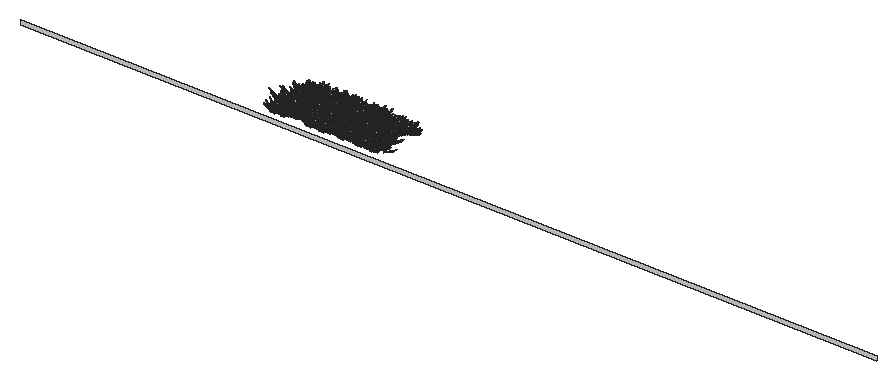
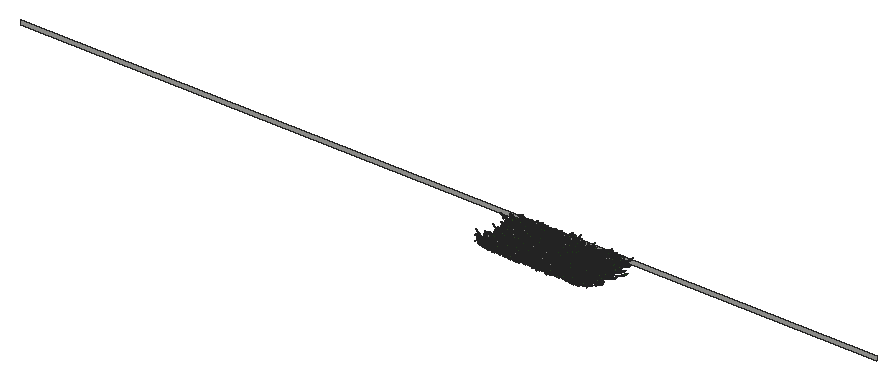
# SketchUp Ruby script. Lengths in inches.
U = 1.inch
M = Sketchup.active_model
def pt(a) = Geom::Point3d.new(a.map { |v| v * U })
def face(e, loops, mat)
  f = e.add_face(loops[0].map { |a| pt(a) })
  loops[1..].each { |l| e.add_face(l.map { |a| pt(a) }).erase! }
  f.material = f.back_material = mat if mat
  f
end
# faces: each face lists its corners as indices into pts; further lists are holes
def faces(e, pts, list, mat = nil) = list.each { |f| face(e, (f[0].is_a?(Array) ? f : [f]).map { |l| l.map { |i| pts[i] } }, mat) }
# xy, xz, yz: faces in a plane at the given z, y or x. An outline is a flat list of corners, or four numbers for a rectangle; further outlines are holes
def ring(l) = l.size == 4 ? [[l[0], l[1]], [l[2], l[1]], [l[2], l[3]], [l[0], l[3]]] : l.each_slice(2).to_a
def flat(e, list, mat, &to3) = list.each { |f| face(e, (f[0].is_a?(Array) ? f : [f]).map { |l| ring(l).map { |u, v| to3.(u, v) } }, mat) }
def xy(e, z, list, mat = nil) = flat(e, list, mat) { |x, y| [x, y, z] }
def xz(e, y, list, mat = nil) = flat(e, list, mat) { |x, z| [x, y, z] }
def yz(e, x, list, mat = nil) = flat(e, list, mat) { |y, z| [x, y, z] }
def lines(e, pts, list) = list.each { |a, b| e.add_line(pt(pts[a]), pt(pts[b])) }
# prism: a flat outline (further loops are holes) pulled along v
def prism(e, loops, v, mat = nil)
  f = face(e, loops, mat); d = Geom::Vector3d.new(v.map { |x| x * U })
  f.pushpull(f.normal.samedirection?(d) ? d.length : -d.length)
end
def box(e, o, s, mat = nil) = prism(e, [[o, [o[0] + s[0], o[1], o[2]], [o[0] + s[0], o[1] + s[1], o[2]], [o[0], o[1] + s[1], o[2]]]], [0, 0, s[2]], mat)
def at(x, y, z, deg = 0) = Geom::Transformation.translation(pt([x, y, z])) * Geom::Transformation.rotation(ORIGIN, Z_AXIS, deg.degrees)
def axes(o, x, y, z) = Geom::Transformation.new([*x, 0, *y, 0, *z, 0, *pt(o).to_a, 1])
def part(name) = M.definitions.add(name)
# library, detail: a bought-in or finely detailed component or shape, given as its bounding box
def library(name, o, s) = part(name).tap { |d| box(d.entities, o, s) }
def detail(e, o, s) = box(e.add_group.entities, o, s)
def put(e, d, t, mat = nil) = e.add_instance(d, t).tap { |i| i.material = mat if mat }
def group(e, t, mat = nil) = e.add_group.tap { |g| g.transformation = t; g.material = mat if mat }.entities
root = M.entities
M.materials.add("Material82").color = [68, 110, 58]
M.materials.add("Material83").color = [48, 90, 38]
M.materials.add("Material84").color = [68, 110, 48]
M.materials.add("Material85").color = [48, 90, 48]
M.materials.add("Material86").color = [58, 110, 58]
M.materials.add("Material87").color = [58, 90, 38]
M.materials.add("Material88").color = [68, 100, 58]
M.materials.add("Material89").color = [48, 100, 38]
c1 = part("grass00")
p = [[-0.6875,0.15,0],[-0.56,0.08,5.52],[-0.04,0.03,2.76],[0.48,-0.02,0],[0.35,-0.02,5.52],[-0.1,-0.14,5.52],
  [-0.12,0.65,8.37],[-0.42,0.65,8.37]]
faces(c1.entities,p,[[0,1,2,3],[3,2,4],[1,5,2],[5,4,2],[1,6,5],[4,5,6],[7,6,1]])
c2 = part("Group16\#1")
put(c2.entities,c1,axes([1.44,-0.61,-0.01],[0.05352,0.12609,0],[-0.10704,0.04543,0.07239],[0.06664,-0.02828,0.11628]),"Material85")
put(c2.entities,c1,axes([0.76,-0.15,-0.01],[0.04676,0.24062,0],[-0.23162,0.04501,0.06642],[0.0652,-0.01267,0.23595]),"Material82")
put(c2.entities,c1,axes([0.79,0.01,-0.01],[-0.00606,0.34651,0],[-0.34381,-0.00602,0.0432],[0.04319,0.00076,0.34386]))
put(c2.entities,c1,axes([1,0.23,-0.01],[-0.07192,0.31144,0],[-0.28722,-0.06632,0.1236],[0.12043,0.02781,0.29478]),"Material84")
put(c2.entities,c1,axes([1.66,0.77,-0.01],[-0.13828,0.29651,0],[-0.21551,-0.1005,0.22471],[0.20365,0.09498,0.23779]),"Material89")
put(c2.entities,c1,axes([0.6875,0.52,-0.01],[-0.18126,0.24051,0],[-0.22746,-0.17142,0.09788],[0.07817,0.05891,0.28481]),"Material84")
put(c2.entities,c1,axes([0.68,0.78,-0.01],[-0.215,0.18688,0],[-0.12385,-0.14248,0.21334],[0.13995,0.16101,0.18878]),"Material82")
put(c2.entities,c1,axes([0.56,1,-0.01],[-0.13756,0.07624,0],[-0.06159,-0.11112,0.0927],[0.04494,0.08108,0.12705]),"Material84")
put(c2.entities,c1,axes([0.2,0.64,-0.01],[-0.23729,0.07254,0],[-0.05711,-0.18681,0.153],[0.04473,0.14632,0.19535]),"Material89")
put(c2.entities,c1,axes([0.0625,0.72,-0.01],[-0.28874,0.02525,0],[-0.02179,-0.24916,0.14647],[0.01276,0.14591,0.25012]),"Material82")
put(c2.entities,c1,axes([-0.08,0.62,-0.01],[-0.34089,-0.04187,0],[0.03255,-0.26504,0.216],[-0.02633,0.21439,0.26703]),"Material89")
put(c2.entities,c1,axes([-0.34,0.98,-0.01],[-0.14314,-0.0493,0],[0.04397,-0.12769,0.06843],[-0.02228,0.0647,0.13505]),"Material89")
put(c2.entities,c1,axes([-0.87,1.45,-0.01],[-0.23488,-0.14114,0],[0.13761,-0.22901,0.06087],[-0.03135,0.05217,0.26717]))
put(c2.entities,c1,axes([-0.72,0.77,-0.01],[-0.14208,-0.13251,0],[0.07209,-0.0773,0.16301],[-0.11118,0.11922,0.1057]),"Material89")
put(c2.entities,c1,axes([-0.62,0.43,-0.01],[-0.14845,-0.21203,0],[0.18654,-0.13061,0.12304],[-0.10079,0.07057,0.22772]),"Material82")
put(c2.entities,c1,axes([-0.68,0.29,-0.01],[-0.13639,-0.32136,0],[0.31723,-0.13464,0.05579],[-0.05136,0.0218,0.34462]),"Material83")
put(c2.entities,c1,axes([-0.64,0.125,-0.01],[-0.0458,-0.23569,0],[0.22124,-0.043,0.08276],[-0.08124,0.01579,0.22538]),"Material86")
put(c2.entities,c1,axes([-1.6,-0.03,-0.01],[0.00576,-0.32897,0],[0.27526,0.00482,0.18018],[-0.18015,-0.00315,0.2753]),"Material84")
put(c2.entities,c1,axes([-1.36,-0.31,-0.01],[0.05718,-0.24765,0],[0.18172,0.04196,0.17267],[-0.16825,-0.03885,0.1865]),"Material89")
put(c2.entities,c1,axes([-1.54,-0.72,-0.01],[0.06537,-0.14017,0],[0.13555,0.06321,0.03939],[-0.0357,-0.01665,0.14956]))
put(c2.entities,c1,axes([-1.19,-0.9,-0.01],[0.09597,-0.12735,0],[0.11214,0.08451,0.07557],[-0.06035,-0.04548,0.14042]),"Material88")
put(c2.entities,c1,axes([-0.47,-0.54,-0.01],[0.11588,-0.10072,0],[0.0618,0.0711,0.12124],[-0.07953,-0.0915,0.0942]))
put(c2.entities,c1,axes([-0.47,-0.84,-0.01],[0.11927,-0.0661,0],[0.06603,0.11913,0.00646],[-0.00313,-0.00565,0.13621]),"Material84")
put(c2.entities,c1,axes([-0.38,-1.24,-0.01],[0.28037,-0.08571,0],[0.0618,0.20215,0.20315],[-0.05939,-0.19428,0.21139]),"Material88")
put(c2.entities,c1,axes([-0.06,-0.66,-0.01],[0.22719,-0.01987,0],[0.01247,0.14255,0.17758],[-0.01547,-0.17691,0.1431]),"Material87")
put(c2.entities,c1,axes([0.11,-0.89,-0.01],[0.14882,0.01828,0],[-0.01058,0.08611,0.12229],[0.01491,-0.12138,0.08676]),"Material85")
put(c2.entities,c1,axes([0.25,-0.72,-0.01],[0.20481,0.07053,0],[-0.06206,0.18022,0.10291],[0.03351,-0.0973,0.1906]),"Material85")
put(c2.entities,c1,axes([0.85,-1.42,-0.01],[0.16481,0.09904,0],[-0.09472,0.15762,0.05616],[0.02893,-0.04814,0.18389]),"Material84")
put(c2.entities,c1,axes([1.01,-1.09,-0.01],[0.21858,0.20385,0],[-0.17495,0.1876,0.15339],[0.10462,-0.11218,0.25652]),"Material89")
put(c2.entities,c1,axes([1.01,-0.71,-0.01],[0.08733,0.12473,0],[-0.06445,0.04512,0.13037],[0.1068,-0.07477,0.07867]),"Material85")
c3 = part("Group15\#1")
put(c3.entities,c2,at(0,0,0))
c4 = part("3darcstudiotree_grass00\#1")
put(c4.entities,c3,at(0,0,0))
xz(root,273.41,[[486.41,-37.24,1048.66,-34.17]])
put(root,c4,axes([705.16,281.1875,-34.17],[2.17079,-1.3067,0],[3.53732,0.91396,-0.04807],[0.21538,0.05565,1.69791]))
put(root,c4,axes([711.01,281.2,-34.17],[4.07054,-0.47424,0],[1.26442,1.68794,-0.05518],[0.08285,0.1106,1.77288]))
put(root,c4,axes([650.73,281.26,-34.17],[0.55958,-1.81201,0],[3.80263,0.18264,-0.0324],[0.16574,0.00796,1.47946]))
put(root,c4,axes([674.03,281.33,-34.17],[1.12764,-1.73077,0],[4.18377,0.42395,-0.01129],[0.06303,0.00639,1.86628]))
put(root,c4,axes([695.42,281.47,-34.17],[1.22394,-1.54587,0],[4.34445,0.53497,-0.04262],[0.21661,0.02667,1.81655]))
put(root,c4,axes([683.82,281.62,-34.17],[-3.03372,-1.40875,0],[3.08967,-1.03482,-0.05304],[0.26,-0.08708,1.95407]))
put(root,c4,axes([678.8,282.65,-34.17],[1.40551,-1.64885,0],[4.26228,0.56508,-0.02131],[0.10181,0.0135,1.69918]))
put(root,c4,axes([683.02,282.95,-34.17],[1.31732,-1.5277,0],[3.94533,0.52911,-0.01889],[0.1126,0.0151,1.96679]))
put(root,c4,axes([706.14,283.05,-34.17],[1.63405,-1.64828,0],[3.24927,0.50099,-0.00888],[0.05923,0.00913,1.87213]))
put(root,c4,axes([652.69,282.59,-34.17],[-3.98203,-0.87024,0],[2.1917,-1.55976,-0.02403],[0.066,-0.04697,1.92026]))
put(root,c4,axes([699.89,282.77,-34.17],[-3.61082,-0.39433,0],[1.20081,-1.71014,-0.02644],[0.03989,-0.05681,1.9068]))
put(root,c4,axes([662.19,282.87,-34.17],[-3.87962,-0.67736,0],[1.4284,-1.27243,-0.0129],[0.02606,-0.02321,1.31952]))
put(root,c4,axes([697.15,283.12,-34.17],[3.46015,0.38109,0],[-0.88814,1.25417,-0.03829],[-0.05842,0.0825,1.40372]))
put(root,c4,axes([692.47,282.8,-34.17],[-3.41936,-0.32293,0],[0.80872,-1.33182,-0.00326],[0.00565,-0.00931,1.93944]))
put(root,c4,axes([674.8,283.16,-34.17],[3.02481,0.98705,0],[-2.84435,1.35567,-0.00662],[-0.02068,0.00986,1.63949]))
put(root,c4,axes([670.36,283.8,-34.17],[0.88446,1.28365,0],[-3.4154,0.366,-0.02204],[-0.14997,0.01607,1.87051]))
put(root,c4,axes([656.75,283.9,-34.17],[-0.33098,1.70392,0],[-3.92143,-0.11847,-0.03234],[-0.20787,-0.00628,1.90052]))
put(root,c4,axes([656.83,284.73,-34.17],[4.23456,-0.44217,0],[1.03247,1.53783,-0.03329],[0.03822,0.05692,1.35616]))
put(root,c4,axes([705.21,284.58,-34.17],[-1.01765,1.47435,0],[-4.56253,-0.4898,-0.0223],[-0.09653,-0.01036,1.58974]))
put(root,c4,axes([664.13,284.81,-34.17],[0.47172,1.49628,0],[-3.52699,0.17294,-0.00588],[-0.02991,0.00147,1.36568]))
put(root,c4,axes([712.59,285.43,-34.17],[0.9992,-1.70874,0],[3.78612,0.34433,-0.00305],[0.01806,0.00164,1.76865]))
put(root,c4,axes([686.77,285.14,-34.17],[-3.90096,-0.14279,0],[0.42836,-1.82008,-0.06502],[0.0247,-0.10495,1.42798]))
put(root,c4,axes([700.77,285.56,-34.17],[4.57837,0.42186,0],[-0.79113,1.33536,-0.04207],[-0.04884,0.08244,1.32997]))
put(root,c4,axes([668.71,285.52,-34.17],[1.5336,1.30723,0],[-4.13356,0.75421,-0.03574],[-0.18177,0.03317,1.91331]))
put(root,c4,axes([673.95,286,-34.17],[3.57543,-0.38769,0],[0.94849,1.36047,-0.03828],[0.05948,0.08532,1.57185]))
put(root,c4,axes([695.66,286.02,-34.17],[3.20776,-0.47754,0],[1.28857,1.34619,-0.04981],[0.10847,0.11332,1.68613]))
put(root,c4,axes([678.26,285.74,-34.17],[0.98392,1.60393,0],[-4.31274,0.41147,-0.01063],[-0.04621,0.00441,1.48723]))
put(root,c4,axes([650.65,286.05,-34.17],[-2.94402,-0.61655,0],[1.96985,-1.46292,-0.05452],[0.11404,-0.08469,1.404]))
put(root,c4,axes([691.23,286.08,-34.17],[-4.29885,0.51765,0],[-1.3445,-1.73657,-0.03433],[-0.03931,-0.05078,1.35329]))
put(root,c4,axes([696.89,286.72,-34.17],[-0.83396,-1.47678,0],[3.24144,-0.28469,-0.00779],[0.04244,-0.00373,1.38852]))
put(root,c4,axes([701.68,287,-34.17],[0.8669,-1.63737,0],[4.38165,0.36081,-0.01659],[0.07514,0.00619,1.55232]))
put(root,c4,axes([686.35,286.9,-34.17],[2.831,1.13552,0],[-3.26481,1.26594,-0.00938],[-0.03813,0.01479,1.95578]))
put(root,c4,axes([679.07,286.87,-34.17],[2.31946,1.24356,0],[-3.54601,1.02866,-0.02079],[-0.06877,0.01995,1.35493]))
put(root,c4,axes([668.67,287.19,-34.17],[3.58882,-0.43849,0],[1.01017,1.28588,-0.04073],[0.06773,0.08621,1.43775]))
put(root,c4,axes([661.73,287.42,-34.17],[3.87508,-0.19158,0],[0.55593,1.74888,-0.03701],[0.02742,0.08626,1.99511]))
put(root,c4,axes([706.78,286.81,-34.17],[-1.66334,1.46333,0],[-4.128,-0.72978,-0.00369],[-0.01567,-0.00277,1.57624]))
put(root,c4,axes([653.03,287.47,-34.17],[-2.23453,-0.97852,0],[2.77364,-0.9851,-0.04825],[0.23755,-0.08437,1.85346]))
put(root,c4,axes([688.76,288.01,-34.17],[0.13943,1.51336,0],[-3.52829,0.05056,-0.04285],[-0.2957,0.00424,1.82733]))
put(root,c4,axes([674.53,287.92,-34.17],[-2.1552,1.3099,0],[-3.57978,-0.91604,-0.05659],[-0.20761,-0.05313,1.39892]))
put(root,c4,axes([657.72,288.18,-34.17],[-3.02099,1.21639,0],[-3.37871,-1.30508,-0.0181],[-0.07062,-0.02728,1.93624]))
put(root,c4,axes([663.9,288.95,-34.17],[4.11072,0.52115,0],[-1.12592,1.38127,-0.00634],[-0.01225,0.01503,1.74238]))
put(root,c4,axes([651.66,289.22,-34.17],[1.39356,-1.72752,0],[4.38256,0.54985,-0.00448],[0.02218,0.00278,1.79011]))
put(root,c4,axes([711.33,289.61,-34.17],[-0.53843,-1.61653,0],[3.48383,-0.18047,-0.04534],[0.27707,-0.01435,1.62314]))
put(root,c4,axes([706.55,289.17,-34.17],[-1.88196,1.3957,0],[-3.10758,-0.65171,-0.04799],[-0.32006,-0.06712,1.99284]))
put(root,c4,axes([656.34,289.95,-34.17],[0.57397,-1.69302,0],[4.41794,0.23295,-0.0102],[0.05353,0.00282,1.76846]))
put(root,c4,axes([690.64,289.83,-34.17],[-0.52019,-1.47295,0],[3.61124,-0.19836,-0.01078],[0.07028,-0.00386,1.79898]))
put(root,c4,axes([694.17,289.66,-34.17],[-0.97814,1.51943,0],[-3.80237,-0.3807,-0.01715],[-0.08253,-0.00826,1.46021]))
put(root,c4,axes([675.88,289.77,-34.17],[0.84595,1.74988,0],[-3.45616,0.25986,-0.03349],[-0.2005,0.01508,1.60736]))
put(root,c4,axes([666.96,290,-34.17],[-3.51608,0.58555,0],[-1.76508,-1.64843,-0.01449],[-0.02729,-0.02549,1.64714]))
put(root,c4,axes([702.85,290.39,-34.17],[2.67266,1.37649,0],[-3.28703,0.99263,-0.02004],[-0.06999,0.02114,1.3651]))
put(root,c4,axes([677.375,290.53,-34.17],[-2.74028,-0.81988,0],[2.08475,-1.08371,-0.01586],[0.05642,-0.02933,1.52204]))
put(root,c4,axes([683.625,290.22,-34.17],[-2.48253,1.23787,0],[-2.67891,-0.83558,-0.01059],[-0.04346,-0.01356,1.33934]))
put(root,c4,axes([679.91,291.375,-34.17],[-3.00354,-1.31894,0],[3.37135,-1.19405,-0.05274],[0.22952,-0.08129,1.98669]))
put(root,c4,axes([686.84,291.86,-34.17],[1.37504,-1.64012,0],[4.21946,0.55019,-0.04027],[0.19656,0.02563,1.71232]))
put(root,c4,axes([703.21,292.11,-34.17],[2.76982,-1.52047,0],[2.85461,0.80878,-0.0087],[0.04308,0.01221,1.60603]))
put(root,c4,axes([662.84,292.1875,-34.17],[2.88399,-0.92183,0],[2.75264,1.33938,-0.02341],[0.07157,0.03482,1.59067]))
put(root,c4,axes([674.53,291.59,-34.17],[-4.47684,0.54828,0],[-1.1065,-1.40519,-0.03919],[-0.07055,-0.08959,1.69748]))
put(root,c4,axes([705.33,291.6,-34.17],[-4.11453,0.51388,0],[-1.13165,-1.40923,-0.01419],[-0.02668,-0.03323,1.75006]))
put(root,c4,axes([689.09,291.6875,-34.17],[-4.23608,0.30685,0],[-0.85226,-1.82987,-0.05609],[-0.05564,-0.11947,1.94158]))
put(root,c4,axes([697.05,291.95,-34.17],[2.07706,1.01263,0],[-2.63538,0.84072,-0.02717],[-0.1514,0.0483,1.82093]))
put(root,c4,axes([711.39,291.98,-34.17],[-3.63945,-0.58666,0],[1.30533,-1.25945,-0.04864],[0.1019,-0.09832,1.4319]))
put(root,c4,axes([657.75,292.07,-34.17],[-4.25916,-0.67423,0],[1.26133,-1.23925,-0.04034],[0.09396,-0.09232,1.58691]))
put(root,c4,axes([650.1,291.66,-34.17],[-3.70599,0.79197,0],[-2.20745,-1.60656,-0.0133],[-0.03552,-0.02585,1.94738]))
put(root,c4,axes([666.67,292.51,-34.17],[-4.16919,-0.21002,0],[0.49933,-1.5417,-0.0157],[0.01299,-0.04011,1.92971]))
put(root,c4,axes([651.44,293.28,-34.17],[-0.43315,-1.7077,0],[3.80872,-0.15025,-0.05423],[0.31945,-0.0126,1.69842]))
put(root,c4,axes([673.71,293.84,-34.17],[1.31559,-1.26739,0],[3.71813,0.60026,-0.00546],[0.02236,0.00361,1.33158]))
put(root,c4,axes([685.03,293.35,-34.17],[0.02685,1.39613,0],[-4.67009,0.01397,-0.03677],[-0.14547,0.00044,1.38481]))
put(root,c4,axes([681.34,293.98,-34.17],[2.75881,-1.06303,0],[3.05708,1.23394,-0.03867],[0.14354,0.05794,1.7417]))
put(root,c4,axes([663.39,293.77,-34.17],[-1.10259,-1.32087,0],[4.19794,-0.54501,-0.05688],[0.29749,-0.03862,1.82396]))
put(root,c4,axes([708.83,294.25,-34.17],[0.84647,-1.73268,0],[3.98325,0.30265,-0.00212],[0.01137,0.00086,1.6588]))
put(root,c4,axes([702.01,293.55,-34.17],[-2.78854,1.36928,0],[-2.88748,-0.91457,-0.04358],[-0.20411,-0.06465,1.66757]))
put(root,c4,axes([689.57,294.65,-34.17],[3.75686,0.07381,0],[-0.21994,1.74119,-0.00527],[-0.00126,0.00998,1.59512]))
put(root,c4,axes([655.41,294.69,-34.17],[2.35188,-1.38482,0],[3.12769,0.82614,-0.05113],[0.23612,0.06237,1.56833]))
put(root,c4,axes([695.48,294.06,-34.17],[-2.45653,1.59128,0],[-3.13753,-0.75331,-0.03488],[-0.14833,-0.03561,1.37068]))
put(root,c4,axes([666.9,294.87,-34.17],[0.70204,1.43301,0],[-3.58325,0.27302,-0.03785],[-0.19362,0.01475,1.42505]))
put(root,c4,axes([703.45,296.27,-34.17],[3.07151,-0.57195,0],[1.60637,1.34169,-0.03456],[0.08725,0.07287,1.66747]))
put(root,c4,axes([697.01,296.33,-34.17],[0.41064,-1.32496,0],[4.30887,0.2077,-0.02785],[0.12721,0.00613,1.49696]))
put(root,c4,axes([667.25,296.54,-34.17],[3.86131,0.54377,0],[-1.4335,1.58316,-0.00059],[-0.00108,0.0012,1.74794]))
put(root,c4,axes([664.02,296.25,-34.17],[-3.05685,-0.82947,0],[2.14696,-1.23058,-0.02104],[0.07287,-0.04177,1.73448]))
put(root,c4,axes([678.16,296.72,-34.17],[2.41246,-1.41032,0],[3.04441,0.80995,-0.04469],[0.24595,0.06543,1.8275]))
put(root,c4,axes([685.41,296.81,-34.17],[3.60532,-0.46019,0],[1.33734,1.62954,-0.01611],[0.02411,0.02937,1.58139]))
put(root,c4,axes([675.85,296.47,-34.17],[3.77018,0.78532,0],[-1.755,1.3104,-0.05015],[-0.15166,0.11324,1.82381]))
put(root,c4,axes([691.07,296.2,-34.17],[-0.64515,1.28427,0],[-4.09885,-0.32024,-0.03573],[-0.18751,-0.01465,1.67549]))
put(root,c4,axes([655.21,296.27,-34.17],[-3.1964,-0.45712,0],[1.21547,-1.32188,-0.00444],[0.00788,-0.00857,1.39182]))
put(root,c4,axes([707.52,296.61,-34.17],[-3.33624,1.28886,0],[-2.34327,-0.94338,-0.00183],[-0.00717,-0.00289,1.40539]))
put(root,c4,axes([651.53,296.92,-34.17],[-3.35036,0.87409,0],[-2.07562,-1.23735,-0.03289],[-0.10016,-0.05971,1.55622]))
put(root,c4,axes([662.66,298,-34.17],[2.33049,-1.15129,0],[2.65609,0.83622,-0.01018],[0.04728,0.01488,1.51436]))
put(root,c4,axes([684.76,297.63,-34.17],[2.78328,1.41625,0],[-3.60575,1.10211,-0.03267],[-0.14651,0.04478,1.93988]))
put(root,c4,axes([655.48,297.84,-34.17],[2.67683,1.25305,0],[-2.64635,0.87925,-0.04423],[-0.18001,0.05981,1.38013]))
put(root,c4,axes([651.56,298.33,-34.17],[4.04553,0.2871,0],[-0.83462,1.82911,-0.01866],[-0.01606,0.0352,1.717]))
put(root,c4,axes([700.89,297.9,-34.17],[1.39252,1.41751,0],[-3.18673,0.48689,-0.02409],[-0.14094,0.02153,1.60735]))
put(root,c4,axes([671.94,298.12,-34.17],[-4.2844,-0.03587,0],[0.08793,-1.63328,-0.04949],[0.00646,-0.12004,1.9102]))
put(root,c4,axes([668.9,298.36,-34.17],[-4.02551,-0.90949,0],[2.09135,-1.43967,-0.04075],[0.0999,-0.06877,1.55523]))
put(root,c4,axes([680.73,298.9,-34.17],[4.10034,-0.52862,0],[1.2552,1.51427,-0.04269],[0.08479,0.10229,1.93529]))
put(root,c4,axes([695.04,298.92,-34.17],[3.38301,-0.17676,0],[0.47183,1.40447,-0.04905],[0.03546,0.10554,1.48186]))
put(root,c4,axes([690.97,298.85,-34.17],[2.80686,0.98493,0],[-2.35719,1.04478,-0.00943],[-0.03285,0.01456,1.39243]))
put(root,c4,axes([707.59,298.96,-34.17],[-1.98727,-1.58329,0],[3.14557,-0.61406,-0.01272],[0.05955,-0.01163,1.37453]))
put(root,c4,axes([666.43,299.92,-34.17],[0.60335,-1.83981,0],[4.64218,0.23677,-0.05291],[0.19949,0.01017,1.33374]))
put(root,c4,axes([683.52,299.86,-34.17],[-3.10894,1.29688,0],[-2.64938,-0.9878,-0.02847],[-0.10631,-0.03964,1.40417]))
put(root,c4,axes([663.3,300.61,-34.17],[2.49775,-0.87161,0],[2.87959,1.28342,-0.04815],[0.19249,0.08579,1.9649]))
put(root,c4,axes([702.53,301.15,-34.17],[3.6923,-0.26906,0],[0.83055,1.77269,-0.01263],[0.0116,0.02476,1.73191]))
put(root,c4,axes([708.22,300.86,-34.17],[-2.8282,-0.92386,0],[2.41261,-1.14869,-0.01497],[0.06145,-0.02926,1.82381]))
put(root,c4,axes([694.17,301.11,-34.17],[-1.60359,-1.29455,0],[3.30864,-0.63743,-0.0349],[0.20941,-0.04034,1.84302]))
put(root,c4,axes([672.85,301.23,-34.17],[3.05854,0.58726,0],[-2.04234,1.65433,-0.05845],[-0.11264,0.09124,1.53958]))
put(root,c4,axes([656.625,301.0625,-34.17],[-3.29694,-0.59268,0],[1.38855,-1.20133,-0.0331],[0.08455,-0.07315,1.54531]))
put(root,c4,axes([689.35,301.43,-34.17],[-3.83901,-0.76558,0],[1.48905,-1.16132,-0.0255],[0.09039,-0.0705,1.94297]))
put(root,c4,axes([677.5625,301.18,-34.17],[-1.85089,1.19146,0],[-2.90652,-0.70224,-0.01687],[-0.07661,-0.01851,1.36079]))
put(root,c4,axes([689.25,302.28,-34.17],[3.52935,-0.50726,0],[1.49485,1.61761,-0.06136],[0.11602,0.12555,1.80687]))
put(root,c4,axes([652.26,302.19,-34.17],[-2.79186,-1.03231,0],[2.26214,-0.95152,-0.04465],[0.21173,-0.08906,1.71883]))
put(root,c4,axes([675.62,302.4375,-34.17],[4.31211,0.22009,0],[-0.60247,1.83583,-0.04718],[-0.02535,0.07723,1.4726]))
put(root,c4,axes([711.71,302.75,-34.17],[0.02414,-1.32822,0],[3.48081,0.00984,-0.01704],[0.11733,0.00033,1.79616]))
put(root,c4,axes([678.34,303.14,-34.17],[1.88589,-1.60822,0],[4.27567,0.77981,-0.01],[0.0511,0.00932,1.98774]))
put(root,c4,axes([685.8125,302.54,-34.17],[-0.58657,1.2788,0],[-3.43074,-0.24475,-0.01415],[-0.07642,-0.00545,1.43376]))
put(root,c4,axes([701.84,302.91,-34.17],[4.10063,0.83805,0],[-2.12312,1.61572,-0.0509],[-0.10915,0.08307,1.61215]))
put(root,c4,axes([658.43,303.24,-34.17],[1.13928,-1.32787,0],[4.00016,0.53378,-0.02846],[0.11467,0.0153,1.34635]))
put(root,c4,axes([661.85,303.28,-34.17],[4.20126,0.39077,0],[-0.91213,1.52518,-0.02883],[-0.04091,0.06841,1.84132]))
put(root,c4,axes([696.11,302.92,-34.17],[-2.19345,1.65823,0],[-4.03021,-0.82913,-0.04188],[-0.20563,-0.0423,1.88687]))
put(root,c4,axes([708.21,303.36,-34.17],[2.38559,0.94842,0],[-2.99836,1.17298,-0.03885],[-0.13848,0.05417,1.58937]))
put(root,c4,axes([666.64,303.55,-34.17],[-1.58706,-1.22315,0],[3.88697,-0.78439,-0.02541],[0.09132,-0.01843,1.32108]))
put(root,c4,axes([672.55,304.22,-34.17],[2.23016,-1.08828,0],[2.80047,0.89256,-0.01488],[0.0583,0.01858,1.35946]))
put(root,c4,axes([702.25,304.34,-34.17],[3.39127,-1.14999,0],[2.14538,0.98397,-0.0226],[0.09906,0.04544,1.65792]))
put(root,c4,axes([664.78,304.7,-34.17],[3.24027,-0.98547,0],[2.31887,1.18584,-0.00737],[0.02262,0.01157,1.42978]))
put(root,c4,axes([689.03,304.72,-34.17],[-0.94888,-1.39552,0],[4.53946,-0.48005,-0.04199],[0.20499,-0.02168,1.7807]))
put(root,c4,axes([705.32,305.09,-34.17],[2.51974,-1.17528,0],[3.05999,1.02034,-0.03628],[0.13748,0.04584,1.49031]))
put(root,c4,axes([658.9,305.03,-34.17],[1.43898,-1.34623,0],[3.17438,0.52772,-0.03331],[0.18037,0.02999,1.51731]))
put(root,c4,axes([696.02,304.33,-34.17],[-4.29208,0.36507,0],[-0.8528,-1.5594,-0.00845],[-0.00798,-0.0146,1.35873]))
put(root,c4,axes([650.77,304.67,-34.17],[-3.56566,-0.8896,0],[2.32838,-1.45148,-0.01513],[0.04457,-0.02778,1.79885]))
put(root,c4,axes([679.28,305.03,-34.17],[2.9165,0.98147,0],[-2.52132,1.16527,-0.03219],[-0.13562,0.06268,1.88986]))
put(root,c4,axes([666.375,305.125,-34.17],[2.05839,1.31648,0],[-3.03228,0.73739,-0.00763],[-0.03853,0.00937,1.58363]))
put(root,c4,axes([711.78,305.53,-34.17],[-2.38248,1.06709,0],[-3.21771,-1.11734,-0.02335],[-0.09118,-0.03166,1.67208]))
put(root,c4,axes([685.07,305.62,-34.17],[-3.50072,1.23157,0],[-2.52643,-1.11691,-0.04505],[-0.14682,-0.06491,1.39266]))
put(root,c4,axes([712.45,306.61,-34.17],[2.50615,-1.32245,0],[2.94011,0.86656,-0.03861],[0.1979,0.05833,1.76068]))
put(root,c4,axes([670.31,306.58,-34.17],[1.26993,-1.49927,0],[3.12751,0.41201,-0.03453],[0.23339,0.03075,1.76116]))
put(root,c4,axes([659.06,306.36,-34.17],[1.96702,1.06284,0],[-3.17968,0.91525,-0.05552],[-0.21201,0.06102,1.39481]))
put(root,c4,axes([707.29,306.66,-34.17],[-1.89774,-1.54823,0],[3.70179,-0.70571,-0.04214],[0.19197,-0.0366,1.55921]))
put(root,c4,axes([651.71,306.42,-34.17],[-3.34111,0.18713,0],[-0.56421,-1.56678,-0.00819],[-0.00515,-0.01431,1.3463]))
put(root,c4,axes([701.32,306.93,-34.17],[3.59081,0.56064,0],[-1.39714,1.39174,-0.03237],[-0.06842,0.06816,1.63378]))
put(root,c4,axes([675.62,307.3,-34.17],[2.80865,-0.79423,0],[2.35611,1.29587,-0.04704],[0.15431,0.08487,1.70604]))
put(root,c4,axes([691.71,306.65,-34.17],[-0.90085,1.67926,0],[-4.44806,-0.37112,-0.05558],[-0.25392,-0.02119,1.59125]))
put(root,c4,axes([662.8125,307.52,-34.17],[1.64847,-1.35078,0],[4.23243,0.80334,-0.06017],[0.26789,0.05085,1.73941]))
put(root,c4,axes([686.27,307.15,-34.17],[-4.10859,0.05118,0],[-0.12582,-1.57107,-0.03959],[-0.00691,-0.08629,1.65212]))
put(root,c4,axes([695.7,307.24,-34.17],[-2.91157,1.30067,0],[-2.86972,-0.9991,-0.01581],[-0.05499,-0.01914,1.33135]))
put(root,c4,axes([680.96,307.47,-34.17],[-0.60337,1.5081,0],[-3.83662,-0.23874,-0.0149],[-0.0971,-0.00604,1.9212]))
put(root,c4,axes([712.11,308.59,-34.17],[-1.25473,-1.49042,0],[3.70912,-0.48565,-0.03393],[0.14523,-0.01902,1.3212]))
put(root,c4,axes([662.18,308.67,-34.17],[-4.49573,0.21611,0],[-0.44378,-1.43584,-0.03065],[-0.02667,-0.0863,1.97713]))
put(root,c4,axes([701.48,309.21,-34.17],[-2.33047,-0.97071,0],[3.43186,-1.28143,-0.06171],[0.20646,-0.07709,1.63202]))
put(root,c4,axes([673.39,309.54,-34.17],[4.02075,-0.11832,0],[0.27482,1.45248,-0.02534],[0.01078,0.05696,1.58232]))
put(root,c4,axes([691.98,309.14,-34.17],[1.7612,1.59038,0],[-3.40002,0.5856,-0.01938],[-0.1015,0.01748,1.58937]))
put(root,c4,axes([655.76,309.6875,-34.17],[1.1756,-1.47793,0],[3.44657,0.42639,-0.02865],[0.17647,0.02183,1.74795]))
put(root,c4,axes([708.09,309.15,-34.17],[-3.12054,0.56833,0],[-1.82234,-1.55622,-0.05064],[-0.09583,-0.08183,1.47033]))
put(root,c4,axes([668.95,310.05,-34.17],[2.53276,-1.11904,0],[3.44801,1.21375,-0.02458],[0.09462,0.03331,1.78746]))
put(root,c4,axes([677.39,310.15,-34.17],[3.19182,-1.13301,0],[2.43556,1.06713,-0.02235],[0.10598,0.04644,1.93391]))
put(root,c4,axes([653.24,309.8,-34.17],[2.22198,1.23467,0],[-3.2898,0.92081,-0.0048],[-0.02055,0.00575,1.58899]))
put(root,c4,axes([684.58,309.77,-34.17],[-4.54038,0.15264,0],[-0.30495,-1.41082,-0.04632],[-0.02774,-0.12834,1.89764]))
put(root,c4,axes([694.96,310.17,-34.17],[-4.30049,-0.14117,0],[0.33609,-1.59238,-0.036],[0.01919,-0.09092,1.9513]))
